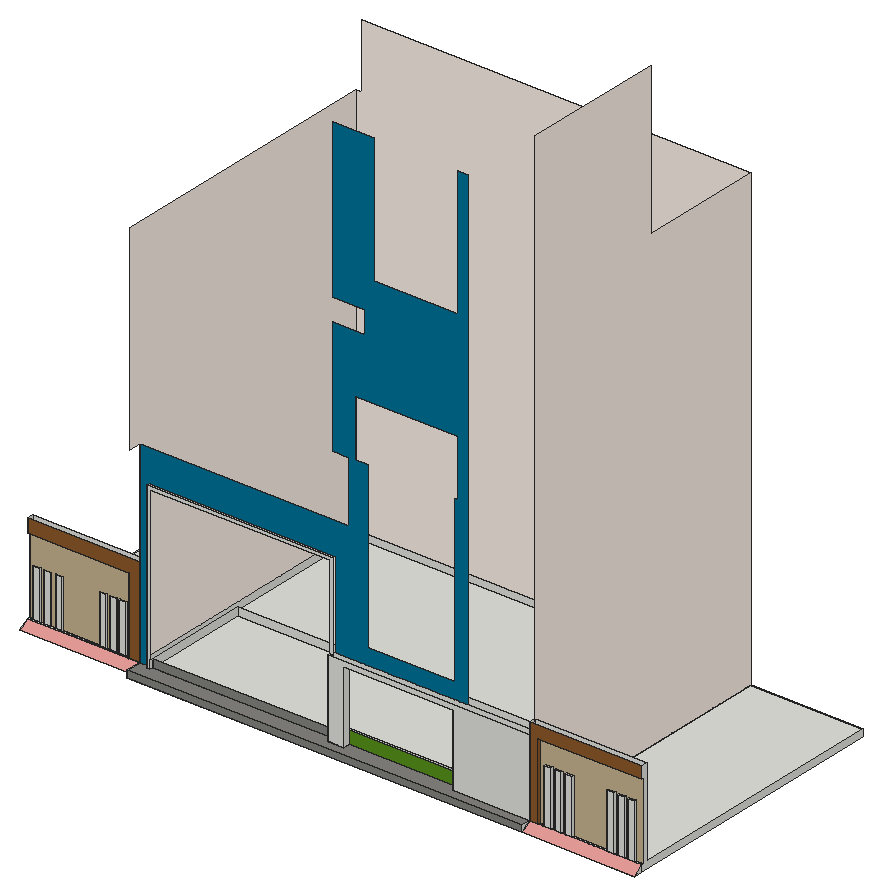
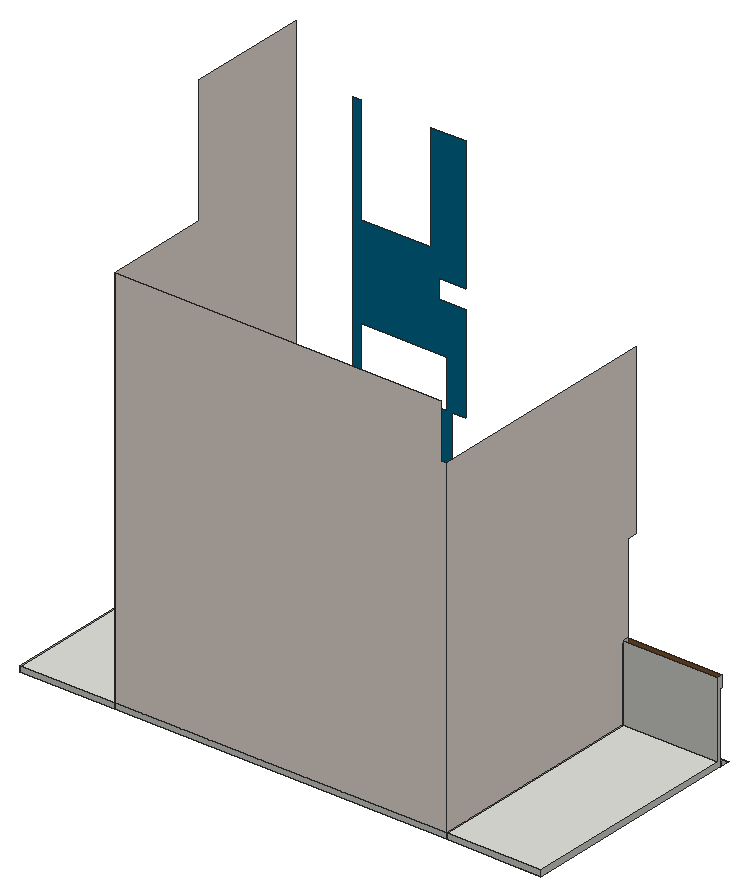
# SketchUp Ruby script. Lengths in inches.
U = 1.inch
M = Sketchup.active_model
def pt(a) = Geom::Point3d.new(a.map { |v| v * U })
def face(e, loops, mat)
  f = e.add_face(loops[0].map { |a| pt(a) })
  loops[1..].each { |l| e.add_face(l.map { |a| pt(a) }).erase! }
  f.material = f.back_material = mat if mat
  f
end
# faces: each face lists its corners as indices into pts; further lists are holes
def faces(e, pts, list, mat = nil) = list.each { |f| face(e, (f[0].is_a?(Array) ? f : [f]).map { |l| l.map { |i| pts[i] } }, mat) }
# xy, xz, yz: faces in a plane at the given z, y or x. An outline is a flat list of corners, or four numbers for a rectangle; further outlines are holes
def ring(l) = l.size == 4 ? [[l[0], l[1]], [l[2], l[1]], [l[2], l[3]], [l[0], l[3]]] : l.each_slice(2).to_a
def flat(e, list, mat, &to3) = list.each { |f| face(e, (f[0].is_a?(Array) ? f : [f]).map { |l| ring(l).map { |u, v| to3.(u, v) } }, mat) }
def xy(e, z, list, mat = nil) = flat(e, list, mat) { |x, y| [x, y, z] }
def xz(e, y, list, mat = nil) = flat(e, list, mat) { |x, z| [x, y, z] }
def yz(e, x, list, mat = nil) = flat(e, list, mat) { |y, z| [x, y, z] }
def lines(e, pts, list) = list.each { |a, b| e.add_line(pt(pts[a]), pt(pts[b])) }
# prism: a flat outline (further loops are holes) pulled along v
def prism(e, loops, v, mat = nil)
  f = face(e, loops, mat); d = Geom::Vector3d.new(v.map { |x| x * U })
  f.pushpull(f.normal.samedirection?(d) ? d.length : -d.length)
end
def box(e, o, s, mat = nil) = prism(e, [[o, [o[0] + s[0], o[1], o[2]], [o[0] + s[0], o[1] + s[1], o[2]], [o[0], o[1] + s[1], o[2]]]], [0, 0, s[2]], mat)
def at(x, y, z, deg = 0) = Geom::Transformation.translation(pt([x, y, z])) * Geom::Transformation.rotation(ORIGIN, Z_AXIS, deg.degrees)
def axes(o, x, y, z) = Geom::Transformation.new([*x, 0, *y, 0, *z, 0, *pt(o).to_a, 1])
def part(name) = M.definitions.add(name)
# library, detail: a bought-in or finely detailed component or shape, given as its bounding box
def library(name, o, s) = part(name).tap { |d| box(d.entities, o, s) }
def detail(e, o, s) = box(e.add_group.entities, o, s)
def put(e, d, t, mat = nil) = e.add_instance(d, t).tap { |i| i.material = mat if mat }
def group(e, t, mat = nil) = e.add_group.tap { |g| g.transformation = t; g.material = mat if mat }.entities
root = M.entities
M.materials.add("[0009_Linen]").color = [250, 240, 230]
M.materials.add("[0034_Wheat]").color = [198, 180, 145]
M.materials.add("[0040_Peru]").color = [140, 90, 43]
M.materials.add("[0097_DeepSkyBlue]").color = [0, 114, 153]
M.materials.add("[Brick Basket]").color = [230, 156, 152]
M.materials.add("[Granite Light Gray]").color = [132, 131, 128]
M.materials.add("[Vegetation Honey Locust]").color = [86, 145, 25]
xy(root,-12,[[420,0,1896,1067.41],[1896,0,2316,36],[0,24,420,60],[1896,36,2316,1067.41],[0,60,0,69,15.39,69,15.39,67,40.95,67,40.95,69,55.2,69,55.2,67,80.76,67,80.76,69,98.33,69,98.33,67,123.89,67,123.89,69,262.89,69,262.89,67,288.45,67,288.45,69,300.83,69,300.83,67,326.39,67,326.39,69,336.83,69,336.83,67,362.39,67,362.39,69,379.38,69,379.38,60],
  [379.38,60,379.38,69,0,69,0,1067.41,420,1067.41,420,60],[15.39,67,40.95,69],[55.2,67,80.76,69],[98.33,67,123.89,69],[262.89,67,288.45,69],
  [300.83,67,326.39,69],[336.83,67,362.39,69]])
xy(root,0,[[1140,36,1200,60]])
xy(root,12,[[1927.54,36,1949.82,43],[1949.82,36,1975.38,43],[1975.38,36,1988.38,43],[1988.38,36,2013.94,43],[2013.94,36,2028.13,43],
  [2028.13,36,2053.69,43],[2053.69,36,2185.76,43],[2185.76,36,2211.32,43],[2211.32,36,2224.38,43],[2224.38,36,2249.94,43],
  [2249.94,36,2262.44,43],[2262.44,36,2288.01,43],[2288.01,36,2316,43],[456,48,468,60],[0,60,379.38,69],
  [468,60,468,455.71,1860,455.71,1860,96,1140,96,1140,60],[1896,60,2316,1067.41],[0,84,420,1067.41]])
xy(root,12,[[420,0,1896,0,1896,36,1608,36,1608,60,1200,60,1200,36,1140,36,1140,60,468,60,468,48,456,48,456,60,420,60]],"[Granite Light Gray]")
xz(root,0,[[420,-12,1896,12]],"[Granite Light Gray]")
xz(root,36,[[1896,-12,2316,12],[1140,0,1200,12],[1140,12,1200,12,1200,280.8,1608,280.8,1608,12,1896,12,1896,300,1140,300],[1949.82,12,1975.38,214.5],[1988.38,12,2013.94,214.5],
  [2028.13,12,2053.69,214.5],[2185.76,12,2211.32,214.5],[2224.38,12,2249.94,214.5],[2262.44,12,2288.01,214.5]])
xz(root,36,[[1896,12,1927.54,12,1927.54,297.5,2316,297.5,2316,342.51,1896,342.51]],"[0040_Peru]")
xz(root,43,[[1949.82,12,1975.38,214.5],[1988.38,12,2013.94,214.5],[2028.13,12,2053.69,214.5],[2185.76,12,2211.32,214.5],[2224.38,12,2249.94,214.5],
  [2262.44,12,2288.01,214.5]])
xz(root,43,[[1927.54,12,1949.82,12,1949.82,214.5,1975.38,214.5,1975.38,12,1988.38,12,1988.38,214.5,2013.94,214.5,2013.94,12,2028.13,12,2028.13,214.5,2053.69,214.5,2053.69,12,2185.76,12,2185.76,214.5,2211.32,214.5,2211.32,12,2224.38,12,2224.38,214.5,2249.94,214.5,2249.94,12,2262.44,12,2262.44,214.5,2288.01,214.5,2288.01,12,2316,12,2316,297.5,1927.54,297.5]],"[0034_Wheat]")
xz(root,48,[[456,12,468,12,468,612,1140,612,1140,300,1152,300,1152,624,456,624]])
xz(root,60,[[0,-12,379.38,12],[379.38,-12,420,12],[1140,0,1140,300,1896,300,1896,0,1608,0,1608,280.8,1200,280.8,1200,0],[1896,12,2316,342.51]])
xz(root,60,[[379.38,12,420,12,420,348,0,348,0,297.5,379.38,297.5]],"[0040_Peru]")
xz(root,60,[[[420,12,456,12,456,624,1152,624,1152,300,1644,300,1644,2076,1608,2076,1608,1598,1296,1598,1296,2076,1140,2076,1140,1488,1260,1488,1260,1404,1140,1404,1140,972,1200,972,1200,744,420,744],[1272,360.11,1272,972,1224,972,1224,1188,1608,1188,1608,972,1596,972,1596,360.11]]],"[0097_DeepSkyBlue]")
xz(root,60,[[468,12,1140,42]],"[Granite Light Gray]")
xz(root,60,[[1200,12,1608,60]],"[Vegetation Honey Locust]")
xz(root,67,[[15.39,-12,40.95,190.5],[55.2,-12,80.76,190.5],[98.33,-12,123.89,190.5],[262.89,-12,288.45,190.5],[300.83,-12,326.39,190.5],
  [336.83,-12,362.39,190.5]])
xz(root,69,[[0,-12,15.39,12],[15.39,-12,40.95,12],[40.95,-12,55.2,12],[55.2,-12,80.76,12],[80.76,-12,98.33,12],
  [98.33,-12,123.89,12],[123.89,-12,262.89,12],[262.89,-12,288.45,12],[288.45,-12,300.83,12],[300.83,-12,326.39,12],
  [326.39,-12,336.83,12],[336.83,-12,362.39,12],[362.39,-12,379.38,12]])
xz(root,69,[[0,12,15.39,12,15.39,190.5,40.95,190.5,40.95,12,55.2,12,55.2,190.5,80.76,190.5,80.76,12,98.33,12,98.33,190.5,123.89,190.5,123.89,12,262.89,12,262.89,190.5,288.45,190.5,288.45,12,300.83,12,300.83,190.5,326.39,190.5,326.39,12,336.83,12,336.83,190.5,362.39,190.5,362.39,12,379.38,12,379.38,297.5,0,297.5]],"[0034_Wheat]")
xz(root,84,[[0,12,420,348]])
xz(root,96,[[1140,12,1200,42],[1200,12,1860,42]])
xz(root,455.71,[[468,12,1860,42]])
xz(root,1067.41,[[0,-12,420,12],[420,-12,1896,12],[1896,-12,2316,12]])
xz(root,1067.41,[[420,12,420,1488,444,1488,444,1728,1896,1728,1896,12]],"[0009_Linen]")
yz(root,0,[[24,-12,60,12,60,-12],[60,-12,69,-11.875],[69,-12,69,297.5,60,297.5,60,348,84,348,84,12,1067.41,12,1067.41,-12],[60,-11.875,69,12]])
yz(root,15.39,[[67,-12,69,190.5]])
yz(root,40.95,[[67,-12,69,190.5]])
yz(root,55.2,[[67,-12,69,190.5]])
yz(root,80.76,[[67,-12,69,190.5]])
yz(root,98.33,[[67,-12,69,190.5]])
yz(root,123.89,[[67,-12,69,190.5]])
yz(root,262.89,[[67,-12,69,190.5]])
yz(root,288.45,[[67,-12,69,190.5]])
yz(root,300.83,[[67,-12,69,190.5]])
yz(root,326.39,[[67,-12,69,190.5]])
yz(root,336.83,[[67,-12,69,190.5]])
yz(root,362.39,[[67,-12,69,190.5]])
yz(root,379.38,[[60,-12,69,12]])
yz(root,379.38,[[60,12,69,297.5]],"[0040_Peru]")
yz(root,420,[[0,-12,0,12,60,12,24,-12],[24,-12,60,12,60,-12],[60,-12,84,348],[84,-12,1067.41,12]])
yz(root,420,[[84,12,84,348,60,348,60,744,12,744,12,1488,1067.41,1488,1067.41,12]],"[0009_Linen]")
yz(root,456,[[48,12,60,624]])
yz(root,468,[[48,12,60,42],[60,12,455.71,42]])
yz(root,1140,[[36,0,60,12],[36,12,60,300],[60,12,96,42]])
yz(root,1200,[[36,0,60,12],[36,12,60,280.8]])
yz(root,1608,[[36,0,60,12],[36,12,60,280.8]])
yz(root,1860,[[96,12,455.71,42]])
yz(root,1896,[[0,-12,36,-12,36,12],[0,-12,36,12,0,12],[36,-12,60,342.51],[60,-12,1067.41,12]])
yz(root,1896,[[60,12,1067.41,12,1067.41,1728,599.71,1728,599.71,2292,60,2292]],"[0009_Linen]")
yz(root,1927.54,[[36,12,43,297.5]],"[0040_Peru]")
yz(root,1949.82,[[36,12,43,214.5]])
yz(root,1975.38,[[36,12,43,214.5]])
yz(root,1988.38,[[36,12,43,214.5]])
yz(root,2013.94,[[36,12,43,214.5]])
yz(root,2028.13,[[36,12,43,214.5]])
yz(root,2053.69,[[36,12,43,214.5]])
yz(root,2185.76,[[36,12,43,214.5]])
yz(root,2211.32,[[36,12,43,214.5]])
yz(root,2224.38,[[36,12,43,214.5]])
yz(root,2249.94,[[36,12,43,214.5]])
yz(root,2262.44,[[36,12,43,214.5]])
yz(root,2288.01,[[36,12,43,214.5]])
yz(root,2316,[[0,-12,36,-12,36,12],[36,-12,1067.41,-12,1067.41,12,60,12,60,342.51,36,342.51,36,297.5,43,297.5,43,12,36,12]])
p = [[2316,0,-12],[2316,36,12],[2288.01,36,12],[2262.44,36,12],[2249.94,36,12],[2224.38,36,12],
  [2211.32,36,12],[2185.76,36,12],[2053.69,36,12],[2028.13,36,12],[2013.94,36,12],[1988.38,36,12],
  [1975.38,36,12],[1949.82,36,12],[1927.54,36,12],[1896,36,12],[1896,0,-12],[420,24,-12],
  [420,60,12],[379.38,60,12],[0,60,12],[0,24,-12],[1896,455.71,12],[1860,455.71,12],
  [468,455.71,12],[420,455.71,12],[1200,96,12],[1200,60,12],[1608,36,0],[1608,0,0],
  [1200,36,0],[1200,0,0],[1140,36,0],[1140,0,0],[1896,60,0],[2316,60,0]]
faces(root,p,[[0,1,2,3,4,5,6,7,8,9,10,11,12,13,14,15,16],[17,18,19,20,21]],"[Brick Basket]")
lines(root,p,[[22,23],[24,25],[26,27],[28,29],[30,31],[32,33],[34,35]])
